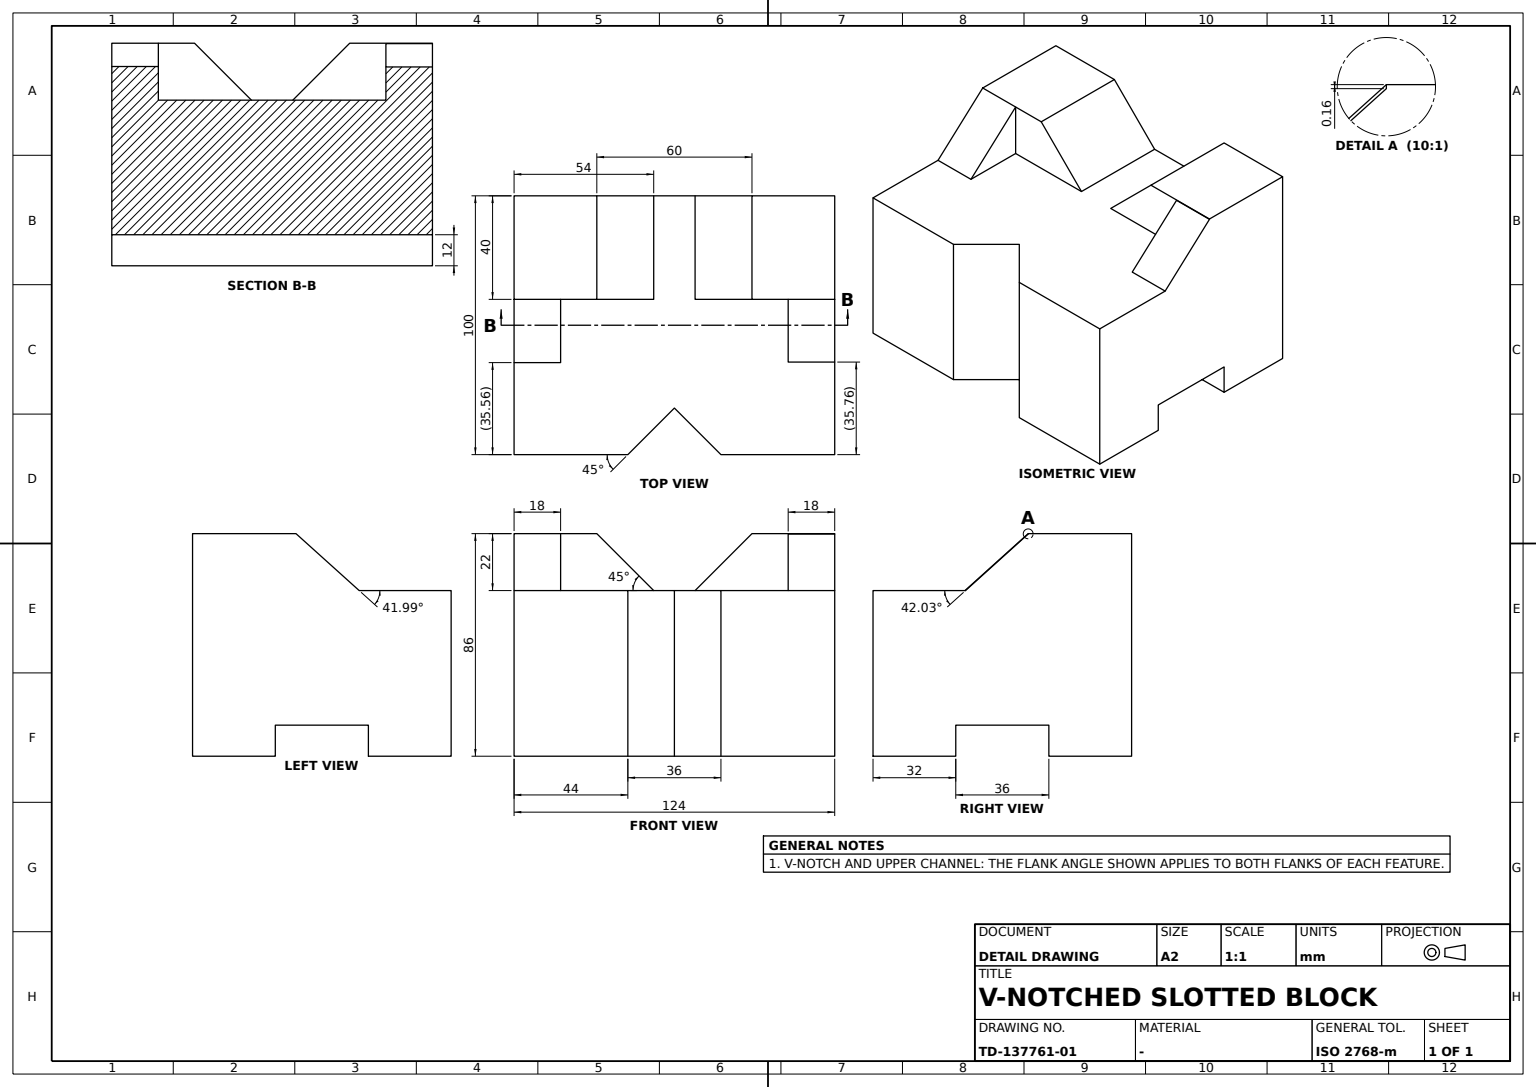
ISO-10303-21;
HEADER;
FILE_DESCRIPTION((''),'2;1');
FILE_NAME('','',(''),(''),'','','');
FILE_SCHEMA(('AUTOMOTIVE_DESIGN'));
ENDSEC;
DATA;
#1=APPLICATION_CONTEXT('');
#2=PRODUCT_CONTEXT('',#1,'mechanical');
#3=PRODUCT('','','',(#2));
#4=PRODUCT_DEFINITION_FORMATION('','',#3);
#5=PRODUCT_DEFINITION_CONTEXT('',#1,'design');
#6=PRODUCT_DEFINITION('','',#4,#5);
#7=PRODUCT_DEFINITION_SHAPE('','',#6);
#8=(LENGTH_UNIT()NAMED_UNIT(*)SI_UNIT(.MILLI.,.METRE.));
#9=(NAMED_UNIT(*)PLANE_ANGLE_UNIT()SI_UNIT($,.RADIAN.));
#10=(NAMED_UNIT(*)SI_UNIT($,.STERADIAN.)SOLID_ANGLE_UNIT());
#11=UNCERTAINTY_MEASURE_WITH_UNIT(LENGTH_MEASURE(1.E-05),#8,'distance_accuracy_value','');
#12=(GEOMETRIC_REPRESENTATION_CONTEXT(3)GLOBAL_UNCERTAINTY_ASSIGNED_CONTEXT((#11))GLOBAL_UNIT_ASSIGNED_CONTEXT((#8,#9,#10))REPRESENTATION_CONTEXT('',''));
#13=CARTESIAN_POINT('',(40.,124.,85.844426));
#14=VERTEX_POINT('',#13);
#15=CARTESIAN_POINT('',(64.235075,124.,64.));
#16=VERTEX_POINT('',#15);
#17=CARTESIAN_POINT('',(52.117538,124.,74.922213));
#18=DIRECTION('',(0.742793172,0.,-0.669520951));
#19=VECTOR('',#18,1000.);
#20=LINE('',#17,#19);
#21=EDGE_CURVE('',#14,#16,#20,.T.);
#22=ORIENTED_EDGE('',*,*,#21,.F.);
#23=CARTESIAN_POINT('',(40.,106.,85.844426));
#24=VERTEX_POINT('',#23);
#25=CARTESIAN_POINT('',(40.,115.,85.844426));
#26=DIRECTION('',(0.,-1.,0.));
#27=VECTOR('',#26,1000.);
#28=LINE('',#25,#27);
#29=EDGE_CURVE('',#14,#24,#28,.T.);
#30=ORIENTED_EDGE('',*,*,#29,.T.);
#31=CARTESIAN_POINT('',(64.235075,106.,64.));
#32=VERTEX_POINT('',#31);
#33=CARTESIAN_POINT('',(52.117538,106.,74.922213));
#34=LINE('',#33,#19);
#35=EDGE_CURVE('',#24,#32,#34,.T.);
#36=ORIENTED_EDGE('',*,*,#35,.T.);
#37=CARTESIAN_POINT('',(64.235075,115.,64.));
#38=LINE('',#37,#27);
#39=EDGE_CURVE('',#16,#32,#38,.T.);
#40=ORIENTED_EDGE('',*,*,#39,.F.);
#41=EDGE_LOOP('',(#22,#30,#36,#40));
#42=FACE_OUTER_BOUND('',#41,.T.);
#43=CARTESIAN_POINT('',(100.,124.,31.763077));
#44=DIRECTION('',(0.669520951,0.,0.742793172));
#45=DIRECTION('',(-0.742793172,0.,0.669520951));
#46=AXIS2_PLACEMENT_3D('',#43,#44,#45);
#47=PLANE('',#46);
#48=ADVANCED_FACE('',(#42),#47,.T.);
#49=CARTESIAN_POINT('',(68.,0.,0.));
#50=VERTEX_POINT('',#49);
#51=CARTESIAN_POINT('',(68.,0.,12.));
#52=VERTEX_POINT('',#51);
#53=CARTESIAN_POINT('',(68.,0.,6.));
#54=DIRECTION('',(0.,0.,1.));
#55=VECTOR('',#54,1000.);
#56=LINE('',#53,#55);
#57=EDGE_CURVE('',#50,#52,#56,.T.);
#58=ORIENTED_EDGE('',*,*,#57,.F.);
#59=CARTESIAN_POINT('',(100.,0.,0.));
#60=VERTEX_POINT('',#59);
#61=CARTESIAN_POINT('',(84.,0.,0.));
#62=DIRECTION('',(1.,0.,0.));
#63=VECTOR('',#62,1000.);
#64=LINE('',#61,#63);
#65=EDGE_CURVE('',#50,#60,#64,.T.);
#66=ORIENTED_EDGE('',*,*,#65,.T.);
#67=CARTESIAN_POINT('',(100.,0.,64.));
#68=VERTEX_POINT('',#67);
#69=CARTESIAN_POINT('',(100.,0.,32.));
#70=LINE('',#69,#55);
#71=EDGE_CURVE('',#60,#68,#70,.T.);
#72=ORIENTED_EDGE('',*,*,#71,.T.);
#73=CARTESIAN_POINT('',(64.444444,0.,64.));
#74=VERTEX_POINT('',#73);
#75=CARTESIAN_POINT('',(82.222222,0.,64.));
#76=LINE('',#75,#63);
#77=EDGE_CURVE('',#74,#68,#76,.T.);
#78=ORIENTED_EDGE('',*,*,#77,.F.);
#79=CARTESIAN_POINT('',(40.,0.,86.));
#80=VERTEX_POINT('',#79);
#81=CARTESIAN_POINT('',(52.222222,0.,75.));
#82=DIRECTION('',(-0.743294146,0.,0.668964732));
#83=VECTOR('',#82,1000.);
#84=LINE('',#81,#83);
#85=EDGE_CURVE('',#74,#80,#84,.T.);
#86=ORIENTED_EDGE('',*,*,#85,.T.);
#87=CARTESIAN_POINT('',(0.,0.,86.));
#88=VERTEX_POINT('',#87);
#89=CARTESIAN_POINT('',(20.,0.,86.));
#90=LINE('',#89,#63);
#91=EDGE_CURVE('',#88,#80,#90,.T.);
#92=ORIENTED_EDGE('',*,*,#91,.F.);
#93=CARTESIAN_POINT('',(0.,0.,0.));
#94=VERTEX_POINT('',#93);
#95=CARTESIAN_POINT('',(0.,0.,43.));
#96=LINE('',#95,#55);
#97=EDGE_CURVE('',#94,#88,#96,.T.);
#98=ORIENTED_EDGE('',*,*,#97,.F.);
#99=CARTESIAN_POINT('',(32.,0.,0.));
#100=VERTEX_POINT('',#99);
#101=CARTESIAN_POINT('',(16.,0.,0.));
#102=LINE('',#101,#63);
#103=EDGE_CURVE('',#94,#100,#102,.T.);
#104=ORIENTED_EDGE('',*,*,#103,.T.);
#105=CARTESIAN_POINT('',(32.,0.,12.));
#106=VERTEX_POINT('',#105);
#107=CARTESIAN_POINT('',(32.,0.,6.));
#108=DIRECTION('',(0.,0.,-1.));
#109=VECTOR('',#108,1000.);
#110=LINE('',#107,#109);
#111=EDGE_CURVE('',#106,#100,#110,.T.);
#112=ORIENTED_EDGE('',*,*,#111,.F.);
#113=CARTESIAN_POINT('',(50.,0.,12.));
#114=DIRECTION('',(-1.,0.,0.));
#115=VECTOR('',#114,1000.);
#116=LINE('',#113,#115);
#117=EDGE_CURVE('',#52,#106,#116,.T.);
#118=ORIENTED_EDGE('',*,*,#117,.F.);
#119=EDGE_LOOP('',(#58,#66,#72,#78,#86,#92,#98,#104,#112,#118));
#120=FACE_OUTER_BOUND('',#119,.T.);
#121=AXIS2_PLACEMENT_3D('',#93,#26,#62);
#122=PLANE('',#121);
#123=ADVANCED_FACE('',(#120),#122,.T.);
#124=CARTESIAN_POINT('',(82.,62.,0.));
#125=VERTEX_POINT('',#124);
#126=CARTESIAN_POINT('',(100.,80.,0.));
#127=VERTEX_POINT('',#126);
#128=CARTESIAN_POINT('',(91.,71.,0.));
#129=DIRECTION('',(0.707106781,0.707106781,0.));
#130=VECTOR('',#129,1000.);
#131=LINE('',#128,#130);
#132=EDGE_CURVE('',#125,#127,#131,.T.);
#133=ORIENTED_EDGE('',*,*,#132,.T.);
#134=CARTESIAN_POINT('',(100.,80.,64.));
#135=VERTEX_POINT('',#134);
#136=CARTESIAN_POINT('',(100.,80.,32.));
#137=LINE('',#136,#55);
#138=EDGE_CURVE('',#127,#135,#137,.T.);
#139=ORIENTED_EDGE('',*,*,#138,.T.);
#140=CARTESIAN_POINT('',(82.,62.,64.));
#141=VERTEX_POINT('',#140);
#142=CARTESIAN_POINT('',(91.,71.,64.));
#143=LINE('',#142,#130);
#144=EDGE_CURVE('',#141,#135,#143,.T.);
#145=ORIENTED_EDGE('',*,*,#144,.F.);
#146=CARTESIAN_POINT('',(82.,62.,32.));
#147=LINE('',#146,#55);
#148=EDGE_CURVE('',#125,#141,#147,.T.);
#149=ORIENTED_EDGE('',*,*,#148,.F.);
#150=EDGE_LOOP('',(#133,#139,#145,#149));
#151=FACE_OUTER_BOUND('',#150,.T.);
#152=DIRECTION('',(0.707106781,-0.707106781,0.));
#153=AXIS2_PLACEMENT_3D('',#124,#152,#129);
#154=PLANE('',#153);
#155=ADVANCED_FACE('',(#151),#154,.T.);
#156=ORIENTED_EDGE('',*,*,#103,.F.);
#157=CARTESIAN_POINT('',(0.,124.,0.));
#158=VERTEX_POINT('',#157);
#159=CARTESIAN_POINT('',(0.,62.,0.));
#160=LINE('',#159,#27);
#161=EDGE_CURVE('',#158,#94,#160,.T.);
#162=ORIENTED_EDGE('',*,*,#161,.F.);
#163=CARTESIAN_POINT('',(32.,124.,0.));
#164=VERTEX_POINT('',#163);
#165=CARTESIAN_POINT('',(16.,124.,0.));
#166=LINE('',#165,#115);
#167=EDGE_CURVE('',#164,#158,#166,.T.);
#168=ORIENTED_EDGE('',*,*,#167,.F.);
#169=CARTESIAN_POINT('',(32.,62.,0.));
#170=DIRECTION('',(0.,1.,0.));
#171=VECTOR('',#170,1000.);
#172=LINE('',#169,#171);
#173=EDGE_CURVE('',#100,#164,#172,.T.);
#174=ORIENTED_EDGE('',*,*,#173,.F.);
#175=EDGE_LOOP('',(#156,#162,#168,#174));
#176=FACE_OUTER_BOUND('',#175,.T.);
#177=AXIS2_PLACEMENT_3D('',#93,#54,#170);
#178=PLANE('',#177);
#179=ADVANCED_FACE('',(#176),#178,.F.);
#180=CARTESIAN_POINT('',(64.444444,18.,64.));
#181=VERTEX_POINT('',#180);
#182=CARTESIAN_POINT('',(40.,18.,86.));
#183=VERTEX_POINT('',#182);
#184=CARTESIAN_POINT('',(52.222222,18.,75.));
#185=LINE('',#184,#83);
#186=EDGE_CURVE('',#181,#183,#185,.T.);
#187=ORIENTED_EDGE('',*,*,#186,.T.);
#188=CARTESIAN_POINT('',(40.,9.,86.));
#189=LINE('',#188,#171);
#190=EDGE_CURVE('',#80,#183,#189,.T.);
#191=ORIENTED_EDGE('',*,*,#190,.F.);
#192=ORIENTED_EDGE('',*,*,#85,.F.);
#193=CARTESIAN_POINT('',(64.444444,9.,64.));
#194=LINE('',#193,#171);
#195=EDGE_CURVE('',#74,#181,#194,.T.);
#196=ORIENTED_EDGE('',*,*,#195,.T.);
#197=EDGE_LOOP('',(#187,#191,#192,#196));
#198=FACE_OUTER_BOUND('',#197,.T.);
#199=DIRECTION('',(-0.668964732,0.,-0.743294146));
#200=AXIS2_PLACEMENT_3D('',#69,#199,#82);
#201=PLANE('',#200);
#202=ADVANCED_FACE('',(#198),#201,.F.);
#203=ORIENTED_EDGE('',*,*,#111,.T.);
#204=ORIENTED_EDGE('',*,*,#173,.T.);
#205=CARTESIAN_POINT('',(32.,124.,12.));
#206=VERTEX_POINT('',#205);
#207=CARTESIAN_POINT('',(32.,124.,6.));
#208=LINE('',#207,#55);
#209=EDGE_CURVE('',#164,#206,#208,.T.);
#210=ORIENTED_EDGE('',*,*,#209,.T.);
#211=CARTESIAN_POINT('',(32.,62.,12.));
#212=LINE('',#211,#171);
#213=EDGE_CURVE('',#106,#206,#212,.T.);
#214=ORIENTED_EDGE('',*,*,#213,.F.);
#215=EDGE_LOOP('',(#203,#204,#210,#214));
#216=FACE_OUTER_BOUND('',#215,.T.);
#217=AXIS2_PLACEMENT_3D('',#105,#62,#108);
#218=PLANE('',#217);
#219=ADVANCED_FACE('',(#216),#218,.T.);
#220=ORIENTED_EDGE('',*,*,#209,.F.);
#221=ORIENTED_EDGE('',*,*,#167,.T.);
#222=CARTESIAN_POINT('',(0.,124.,86.));
#223=VERTEX_POINT('',#222);
#224=CARTESIAN_POINT('',(0.,124.,43.));
#225=LINE('',#224,#55);
#226=EDGE_CURVE('',#158,#223,#225,.T.);
#227=ORIENTED_EDGE('',*,*,#226,.T.);
#228=CARTESIAN_POINT('',(40.,124.,86.));
#229=VERTEX_POINT('',#228);
#230=CARTESIAN_POINT('',(20.,124.,86.));
#231=LINE('',#230,#63);
#232=EDGE_CURVE('',#223,#229,#231,.T.);
#233=ORIENTED_EDGE('',*,*,#232,.T.);
#234=CARTESIAN_POINT('',(40.,124.,85.922213));
#235=LINE('',#234,#109);
#236=EDGE_CURVE('',#229,#14,#235,.T.);
#237=ORIENTED_EDGE('',*,*,#236,.T.);
#238=ORIENTED_EDGE('',*,*,#21,.T.);
#239=CARTESIAN_POINT('',(100.,124.,64.));
#240=VERTEX_POINT('',#239);
#241=CARTESIAN_POINT('',(82.117538,124.,64.));
#242=LINE('',#241,#115);
#243=EDGE_CURVE('',#240,#16,#242,.T.);
#244=ORIENTED_EDGE('',*,*,#243,.F.);
#245=CARTESIAN_POINT('',(100.,124.,0.));
#246=VERTEX_POINT('',#245);
#247=CARTESIAN_POINT('',(100.,124.,32.));
#248=LINE('',#247,#55);
#249=EDGE_CURVE('',#246,#240,#248,.T.);
#250=ORIENTED_EDGE('',*,*,#249,.F.);
#251=CARTESIAN_POINT('',(68.,124.,0.));
#252=VERTEX_POINT('',#251);
#253=CARTESIAN_POINT('',(84.,124.,0.));
#254=LINE('',#253,#115);
#255=EDGE_CURVE('',#246,#252,#254,.T.);
#256=ORIENTED_EDGE('',*,*,#255,.T.);
#257=CARTESIAN_POINT('',(68.,124.,12.));
#258=VERTEX_POINT('',#257);
#259=CARTESIAN_POINT('',(68.,124.,6.));
#260=LINE('',#259,#55);
#261=EDGE_CURVE('',#252,#258,#260,.T.);
#262=ORIENTED_EDGE('',*,*,#261,.T.);
#263=CARTESIAN_POINT('',(50.,124.,12.));
#264=LINE('',#263,#63);
#265=EDGE_CURVE('',#206,#258,#264,.T.);
#266=ORIENTED_EDGE('',*,*,#265,.F.);
#267=EDGE_LOOP('',(#220,#221,#227,#233,#237,#238,#244,#250,#256,#262,#266));
#268=FACE_OUTER_BOUND('',#267,.T.);
#269=AXIS2_PLACEMENT_3D('',#245,#170,#114);
#270=PLANE('',#269);
#271=ADVANCED_FACE('',(#268),#270,.T.);
#272=CARTESIAN_POINT('',(40.,32.,86.));
#273=VERTEX_POINT('',#272);
#274=CARTESIAN_POINT('',(40.,54.,64.));
#275=VERTEX_POINT('',#274);
#276=CARTESIAN_POINT('',(40.,43.,75.));
#277=DIRECTION('',(0.,0.707106781,-0.707106781));
#278=VECTOR('',#277,1000.);
#279=LINE('',#276,#278);
#280=EDGE_CURVE('',#273,#275,#279,.T.);
#281=ORIENTED_EDGE('',*,*,#280,.F.);
#282=CARTESIAN_POINT('',(40.,25.,86.));
#283=LINE('',#282,#171);
#284=EDGE_CURVE('',#183,#273,#283,.T.);
#285=ORIENTED_EDGE('',*,*,#284,.F.);
#286=CARTESIAN_POINT('',(40.,18.,64.));
#287=VERTEX_POINT('',#286);
#288=CARTESIAN_POINT('',(40.,18.,75.));
#289=LINE('',#288,#109);
#290=EDGE_CURVE('',#183,#287,#289,.T.);
#291=ORIENTED_EDGE('',*,*,#290,.T.);
#292=CARTESIAN_POINT('',(40.,36.,64.));
#293=LINE('',#292,#27);
#294=EDGE_CURVE('',#275,#287,#293,.T.);
#295=ORIENTED_EDGE('',*,*,#294,.F.);
#296=EDGE_LOOP('',(#281,#285,#291,#295));
#297=FACE_OUTER_BOUND('',#296,.T.);
#298=CARTESIAN_POINT('',(40.,0.,0.));
#299=AXIS2_PLACEMENT_3D('',#298,#114,#26);
#300=PLANE('',#299);
#301=ADVANCED_FACE('',(#297),#300,.F.);
#302=CARTESIAN_POINT('',(0.,32.,86.));
#303=VERTEX_POINT('',#302);
#304=CARTESIAN_POINT('',(0.,54.,64.));
#305=VERTEX_POINT('',#304);
#306=CARTESIAN_POINT('',(0.,43.,75.));
#307=LINE('',#306,#278);
#308=EDGE_CURVE('',#303,#305,#307,.T.);
#309=ORIENTED_EDGE('',*,*,#308,.F.);
#310=CARTESIAN_POINT('',(20.,32.,86.));
#311=LINE('',#310,#63);
#312=EDGE_CURVE('',#303,#273,#311,.T.);
#313=ORIENTED_EDGE('',*,*,#312,.T.);
#314=ORIENTED_EDGE('',*,*,#280,.T.);
#315=CARTESIAN_POINT('',(20.,54.,64.));
#316=LINE('',#315,#63);
#317=EDGE_CURVE('',#305,#275,#316,.T.);
#318=ORIENTED_EDGE('',*,*,#317,.F.);
#319=EDGE_LOOP('',(#309,#313,#314,#318));
#320=FACE_OUTER_BOUND('',#319,.T.);
#321=CARTESIAN_POINT('',(0.,62.,56.));
#322=DIRECTION('',(0.,0.707106781,0.707106781));
#323=DIRECTION('',(0.,-0.707106781,0.707106781));
#324=AXIS2_PLACEMENT_3D('',#321,#322,#323);
#325=PLANE('',#324);
#326=ADVANCED_FACE('',(#320),#325,.T.);
#327=ORIENTED_EDGE('',*,*,#77,.T.);
#328=CARTESIAN_POINT('',(100.,44.,64.));
#329=VERTEX_POINT('',#328);
#330=CARTESIAN_POINT('',(100.,22.,64.));
#331=LINE('',#330,#171);
#332=EDGE_CURVE('',#68,#329,#331,.T.);
#333=ORIENTED_EDGE('',*,*,#332,.T.);
#334=CARTESIAN_POINT('',(91.,53.,64.));
#335=DIRECTION('',(-0.707106781,0.707106781,0.));
#336=VECTOR('',#335,1000.);
#337=LINE('',#334,#336);
#338=EDGE_CURVE('',#329,#141,#337,.T.);
#339=ORIENTED_EDGE('',*,*,#338,.T.);
#340=ORIENTED_EDGE('',*,*,#144,.T.);
#341=CARTESIAN_POINT('',(100.,102.,64.));
#342=LINE('',#341,#171);
#343=EDGE_CURVE('',#135,#240,#342,.T.);
#344=ORIENTED_EDGE('',*,*,#343,.T.);
#345=ORIENTED_EDGE('',*,*,#243,.T.);
#346=ORIENTED_EDGE('',*,*,#39,.T.);
#347=CARTESIAN_POINT('',(40.,106.,64.));
#348=VERTEX_POINT('',#347);
#349=CARTESIAN_POINT('',(52.117538,106.,64.));
#350=LINE('',#349,#115);
#351=EDGE_CURVE('',#32,#348,#350,.T.);
#352=ORIENTED_EDGE('',*,*,#351,.T.);
#353=CARTESIAN_POINT('',(40.,70.,64.));
#354=VERTEX_POINT('',#353);
#355=CARTESIAN_POINT('',(40.,88.,64.));
#356=LINE('',#355,#27);
#357=EDGE_CURVE('',#348,#354,#356,.T.);
#358=ORIENTED_EDGE('',*,*,#357,.T.);
#359=CARTESIAN_POINT('',(0.,70.,64.));
#360=VERTEX_POINT('',#359);
#361=CARTESIAN_POINT('',(20.,70.,64.));
#362=LINE('',#361,#63);
#363=EDGE_CURVE('',#360,#354,#362,.T.);
#364=ORIENTED_EDGE('',*,*,#363,.F.);
#365=CARTESIAN_POINT('',(0.,62.,64.));
#366=LINE('',#365,#27);
#367=EDGE_CURVE('',#360,#305,#366,.T.);
#368=ORIENTED_EDGE('',*,*,#367,.T.);
#369=ORIENTED_EDGE('',*,*,#317,.T.);
#370=ORIENTED_EDGE('',*,*,#294,.T.);
#371=CARTESIAN_POINT('',(52.222222,18.,64.));
#372=LINE('',#371,#115);
#373=EDGE_CURVE('',#181,#287,#372,.T.);
#374=ORIENTED_EDGE('',*,*,#373,.F.);
#375=ORIENTED_EDGE('',*,*,#195,.F.);
#376=EDGE_LOOP('',(#327,#333,#339,#340,#344,#345,#346,#352,#358,#364,#368,#369,#370,#374,#375));
#377=FACE_OUTER_BOUND('',#376,.T.);
#378=CARTESIAN_POINT('',(0.,0.,64.));
#379=AXIS2_PLACEMENT_3D('',#378,#54,#170);
#380=PLANE('',#379);
#381=ADVANCED_FACE('',(#377),#380,.T.);
#382=CARTESIAN_POINT('',(68.,62.,12.));
#383=LINE('',#382,#171);
#384=EDGE_CURVE('',#52,#258,#383,.T.);
#385=ORIENTED_EDGE('',*,*,#384,.T.);
#386=ORIENTED_EDGE('',*,*,#261,.F.);
#387=CARTESIAN_POINT('',(68.,62.,0.));
#388=LINE('',#387,#171);
#389=EDGE_CURVE('',#50,#252,#388,.T.);
#390=ORIENTED_EDGE('',*,*,#389,.F.);
#391=ORIENTED_EDGE('',*,*,#57,.T.);
#392=EDGE_LOOP('',(#385,#386,#390,#391));
#393=FACE_OUTER_BOUND('',#392,.T.);
#394=AXIS2_PLACEMENT_3D('',#49,#114,#54);
#395=PLANE('',#394);
#396=ADVANCED_FACE('',(#393),#395,.T.);
#397=CARTESIAN_POINT('',(100.,44.,0.));
#398=VERTEX_POINT('',#397);
#399=CARTESIAN_POINT('',(100.,22.,0.));
#400=LINE('',#399,#171);
#401=EDGE_CURVE('',#60,#398,#400,.T.);
#402=ORIENTED_EDGE('',*,*,#401,.F.);
#403=ORIENTED_EDGE('',*,*,#65,.F.);
#404=ORIENTED_EDGE('',*,*,#389,.T.);
#405=ORIENTED_EDGE('',*,*,#255,.F.);
#406=CARTESIAN_POINT('',(100.,102.,0.));
#407=LINE('',#406,#171);
#408=EDGE_CURVE('',#127,#246,#407,.T.);
#409=ORIENTED_EDGE('',*,*,#408,.F.);
#410=ORIENTED_EDGE('',*,*,#132,.F.);
#411=CARTESIAN_POINT('',(91.,53.,0.));
#412=LINE('',#411,#336);
#413=EDGE_CURVE('',#398,#125,#412,.T.);
#414=ORIENTED_EDGE('',*,*,#413,.F.);
#415=EDGE_LOOP('',(#402,#403,#404,#405,#409,#410,#414));
#416=FACE_OUTER_BOUND('',#415,.T.);
#417=ADVANCED_FACE('',(#416),#178,.F.);
#418=ORIENTED_EDGE('',*,*,#401,.T.);
#419=CARTESIAN_POINT('',(100.,44.,32.));
#420=LINE('',#419,#55);
#421=EDGE_CURVE('',#398,#329,#420,.T.);
#422=ORIENTED_EDGE('',*,*,#421,.T.);
#423=ORIENTED_EDGE('',*,*,#332,.F.);
#424=ORIENTED_EDGE('',*,*,#71,.F.);
#425=EDGE_LOOP('',(#418,#422,#423,#424));
#426=FACE_OUTER_BOUND('',#425,.T.);
#427=AXIS2_PLACEMENT_3D('',#59,#62,#170);
#428=PLANE('',#427);
#429=ADVANCED_FACE('',(#426),#428,.T.);
#430=ORIENTED_EDGE('',*,*,#97,.T.);
#431=CARTESIAN_POINT('',(0.,16.,86.));
#432=LINE('',#431,#171);
#433=EDGE_CURVE('',#88,#303,#432,.T.);
#434=ORIENTED_EDGE('',*,*,#433,.T.);
#435=ORIENTED_EDGE('',*,*,#308,.T.);
#436=ORIENTED_EDGE('',*,*,#367,.F.);
#437=CARTESIAN_POINT('',(0.,92.,86.));
#438=VERTEX_POINT('',#437);
#439=CARTESIAN_POINT('',(0.,81.,75.));
#440=VECTOR('',#322,1000.);
#441=LINE('',#439,#440);
#442=EDGE_CURVE('',#360,#438,#441,.T.);
#443=ORIENTED_EDGE('',*,*,#442,.T.);
#444=CARTESIAN_POINT('',(0.,108.,86.));
#445=LINE('',#444,#171);
#446=EDGE_CURVE('',#438,#223,#445,.T.);
#447=ORIENTED_EDGE('',*,*,#446,.T.);
#448=ORIENTED_EDGE('',*,*,#226,.F.);
#449=ORIENTED_EDGE('',*,*,#161,.T.);
#450=EDGE_LOOP('',(#430,#434,#435,#436,#443,#447,#448,#449));
#451=FACE_OUTER_BOUND('',#450,.T.);
#452=AXIS2_PLACEMENT_3D('',#157,#114,#26);
#453=PLANE('',#452);
#454=ADVANCED_FACE('',(#451),#453,.T.);
#455=ORIENTED_EDGE('',*,*,#338,.F.);
#456=ORIENTED_EDGE('',*,*,#421,.F.);
#457=ORIENTED_EDGE('',*,*,#413,.T.);
#458=ORIENTED_EDGE('',*,*,#148,.T.);
#459=EDGE_LOOP('',(#455,#456,#457,#458));
#460=FACE_OUTER_BOUND('',#459,.T.);
#461=AXIS2_PLACEMENT_3D('',#397,#129,#335);
#462=PLANE('',#461);
#463=ADVANCED_FACE('',(#460),#462,.T.);
#464=ORIENTED_EDGE('',*,*,#384,.F.);
#465=ORIENTED_EDGE('',*,*,#117,.T.);
#466=ORIENTED_EDGE('',*,*,#213,.T.);
#467=ORIENTED_EDGE('',*,*,#265,.T.);
#468=EDGE_LOOP('',(#464,#465,#466,#467));
#469=FACE_OUTER_BOUND('',#468,.T.);
#470=AXIS2_PLACEMENT_3D('',#105,#54,#62);
#471=PLANE('',#470);
#472=ADVANCED_FACE('',(#469),#471,.F.);
#473=ORIENTED_EDGE('',*,*,#442,.F.);
#474=ORIENTED_EDGE('',*,*,#363,.T.);
#475=CARTESIAN_POINT('',(40.,92.,86.));
#476=VERTEX_POINT('',#475);
#477=CARTESIAN_POINT('',(40.,81.,75.));
#478=LINE('',#477,#440);
#479=EDGE_CURVE('',#354,#476,#478,.T.);
#480=ORIENTED_EDGE('',*,*,#479,.T.);
#481=CARTESIAN_POINT('',(20.,92.,86.));
#482=LINE('',#481,#63);
#483=EDGE_CURVE('',#438,#476,#482,.T.);
#484=ORIENTED_EDGE('',*,*,#483,.F.);
#485=EDGE_LOOP('',(#473,#474,#480,#484));
#486=FACE_OUTER_BOUND('',#485,.T.);
#487=DIRECTION('',(0.,-0.707106781,-0.707106781));
#488=AXIS2_PLACEMENT_3D('',#437,#323,#487);
#489=PLANE('',#488);
#490=ADVANCED_FACE('',(#486),#489,.T.);
#491=ORIENTED_EDGE('',*,*,#433,.F.);
#492=ORIENTED_EDGE('',*,*,#91,.T.);
#493=ORIENTED_EDGE('',*,*,#190,.T.);
#494=ORIENTED_EDGE('',*,*,#284,.T.);
#495=ORIENTED_EDGE('',*,*,#312,.F.);
#496=EDGE_LOOP('',(#491,#492,#493,#494,#495));
#497=FACE_OUTER_BOUND('',#496,.T.);
#498=AXIS2_PLACEMENT_3D('',#302,#54,#26);
#499=PLANE('',#498);
#500=ADVANCED_FACE('',(#497),#499,.T.);
#501=ORIENTED_EDGE('',*,*,#186,.F.);
#502=ORIENTED_EDGE('',*,*,#373,.T.);
#503=ORIENTED_EDGE('',*,*,#290,.F.);
#504=EDGE_LOOP('',(#501,#502,#503));
#505=FACE_OUTER_BOUND('',#504,.T.);
#506=CARTESIAN_POINT('',(0.,18.,0.));
#507=AXIS2_PLACEMENT_3D('',#506,#26,#62);
#508=PLANE('',#507);
#509=ADVANCED_FACE('',(#505),#508,.F.);
#510=ORIENTED_EDGE('',*,*,#232,.F.);
#511=ORIENTED_EDGE('',*,*,#446,.F.);
#512=ORIENTED_EDGE('',*,*,#483,.T.);
#513=CARTESIAN_POINT('',(40.,108.,86.));
#514=LINE('',#513,#171);
#515=EDGE_CURVE('',#476,#229,#514,.T.);
#516=ORIENTED_EDGE('',*,*,#515,.T.);
#517=EDGE_LOOP('',(#510,#511,#512,#516));
#518=FACE_OUTER_BOUND('',#517,.T.);
#519=ADVANCED_FACE('',(#518),#499,.T.);
#520=CARTESIAN_POINT('',(40.,106.,74.922213));
#521=LINE('',#520,#109);
#522=EDGE_CURVE('',#24,#348,#521,.T.);
#523=ORIENTED_EDGE('',*,*,#522,.F.);
#524=ORIENTED_EDGE('',*,*,#29,.F.);
#525=ORIENTED_EDGE('',*,*,#236,.F.);
#526=ORIENTED_EDGE('',*,*,#515,.F.);
#527=ORIENTED_EDGE('',*,*,#479,.F.);
#528=ORIENTED_EDGE('',*,*,#357,.F.);
#529=EDGE_LOOP('',(#523,#524,#525,#526,#527,#528));
#530=FACE_OUTER_BOUND('',#529,.T.);
#531=ADVANCED_FACE('',(#530),#300,.F.);
#532=ORIENTED_EDGE('',*,*,#522,.T.);
#533=ORIENTED_EDGE('',*,*,#351,.F.);
#534=ORIENTED_EDGE('',*,*,#35,.F.);
#535=EDGE_LOOP('',(#532,#533,#534));
#536=FACE_OUTER_BOUND('',#535,.T.);
#537=CARTESIAN_POINT('',(0.,106.,0.));
#538=AXIS2_PLACEMENT_3D('',#537,#170,#114);
#539=PLANE('',#538);
#540=ADVANCED_FACE('',(#536),#539,.F.);
#541=ORIENTED_EDGE('',*,*,#138,.F.);
#542=ORIENTED_EDGE('',*,*,#408,.T.);
#543=ORIENTED_EDGE('',*,*,#249,.T.);
#544=ORIENTED_EDGE('',*,*,#343,.F.);
#545=EDGE_LOOP('',(#541,#542,#543,#544));
#546=FACE_OUTER_BOUND('',#545,.T.);
#547=ADVANCED_FACE('',(#546),#428,.T.);
#548=CLOSED_SHELL('',(#48,#123,#155,#179,#202,#219,#271,#301,#326,#381,#396,#417,#429,#454,#463,#472,#490,#500,#509,#519,#531,#540,#547));
#549=MANIFOLD_SOLID_BREP('',#548);
#550=ADVANCED_BREP_SHAPE_REPRESENTATION('',(#549),#12);
#551=SHAPE_DEFINITION_REPRESENTATION(#7,#550);
ENDSEC;
END-ISO-10303-21;
